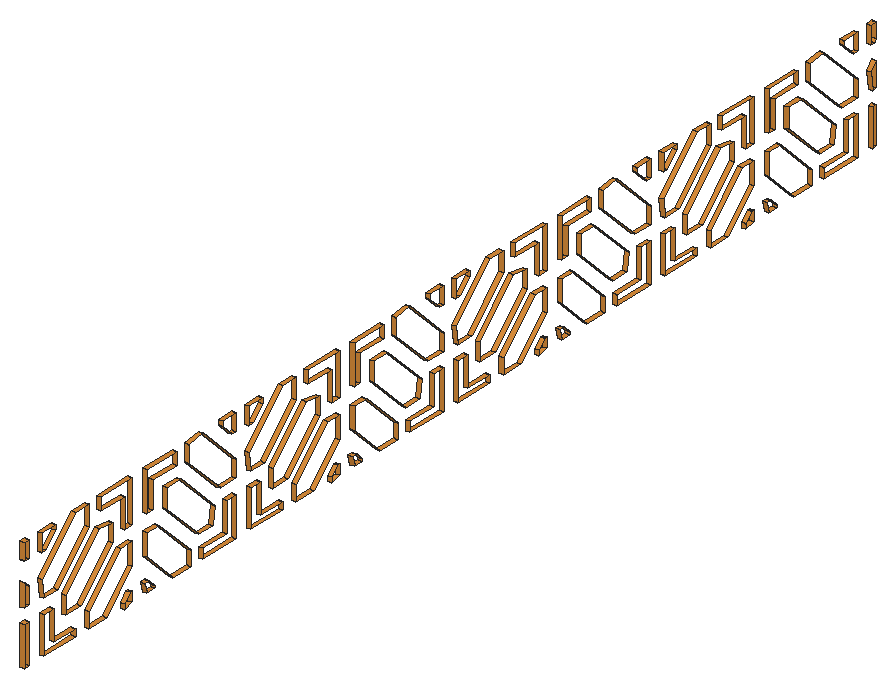
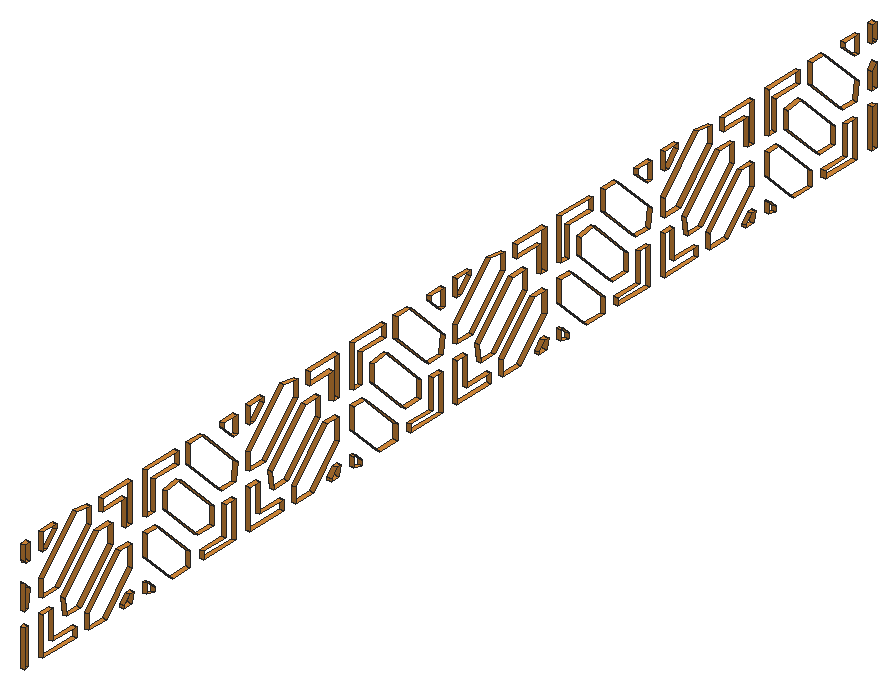
# SketchUp Ruby script. Lengths in inches.
U = 1.inch
M = Sketchup.active_model
def pt(a) = Geom::Point3d.new(a.map { |v| v * U })
def face(e, loops, mat)
  f = e.add_face(loops[0].map { |a| pt(a) })
  loops[1..].each { |l| e.add_face(l.map { |a| pt(a) }).erase! }
  f.material = f.back_material = mat if mat
  f
end
# faces: each face lists its corners as indices into pts; further lists are holes
def faces(e, pts, list, mat = nil) = list.each { |f| face(e, (f[0].is_a?(Array) ? f : [f]).map { |l| l.map { |i| pts[i] } }, mat) }
# xy, xz, yz: faces in a plane at the given z, y or x. An outline is a flat list of corners, or four numbers for a rectangle; further outlines are holes
def ring(l) = l.size == 4 ? [[l[0], l[1]], [l[2], l[1]], [l[2], l[3]], [l[0], l[3]]] : l.each_slice(2).to_a
def flat(e, list, mat, &to3) = list.each { |f| face(e, (f[0].is_a?(Array) ? f : [f]).map { |l| ring(l).map { |u, v| to3.(u, v) } }, mat) }
def xy(e, z, list, mat = nil) = flat(e, list, mat) { |x, y| [x, y, z] }
def xz(e, y, list, mat = nil) = flat(e, list, mat) { |x, z| [x, y, z] }
def yz(e, x, list, mat = nil) = flat(e, list, mat) { |y, z| [x, y, z] }
def lines(e, pts, list) = list.each { |a, b| e.add_line(pt(pts[a]), pt(pts[b])) }
# prism: a flat outline (further loops are holes) pulled along v
def prism(e, loops, v, mat = nil)
  f = face(e, loops, mat); d = Geom::Vector3d.new(v.map { |x| x * U })
  f.pushpull(f.normal.samedirection?(d) ? d.length : -d.length)
end
def box(e, o, s, mat = nil) = prism(e, [[o, [o[0] + s[0], o[1], o[2]], [o[0] + s[0], o[1] + s[1], o[2]], [o[0], o[1] + s[1], o[2]]]], [0, 0, s[2]], mat)
def at(x, y, z, deg = 0) = Geom::Transformation.translation(pt([x, y, z])) * Geom::Transformation.rotation(ORIGIN, Z_AXIS, deg.degrees)
def axes(o, x, y, z) = Geom::Transformation.new([*x, 0, *y, 0, *z, 0, *pt(o).to_a, 1])
def part(name) = M.definitions.add(name)
# library, detail: a bought-in or finely detailed component or shape, given as its bounding box
def library(name, o, s) = part(name).tap { |d| box(d.entities, o, s) }
def detail(e, o, s) = box(e.add_group.entities, o, s)
def put(e, d, t, mat = nil) = e.add_instance(d, t).tap { |i| i.material = mat if mat }
def group(e, t, mat = nil) = e.add_group.tap { |g| g.transformation = t; g.material = mat if mat }.entities
root = M.entities
M.materials.add("1056 AP 9903 Mellow Melon-N").color = [219, 142, 59]
xy(root,171.04,[[14.35,14.79,15.0625,15.84],[14.35,41.6875,15.0625,43.42],[14.35,47.3,15.0625,51.22],[14.35,53.82,15.0625,61.1875],[14.35,87.03,15.0625,88.76],
  [14.35,92.64,15.0625,96.56],[14.35,99.16,15.0625,106.53],[14.35,132.375,15.0625,134.11],[14.35,137.98,15.0625,141.91],[14.35,144.51,15.0625,151.875],
  [14.35,177.72,15.0625,179.45],[14.35,183.33,15.0625,187.25],[14.35,189.85,15.0625,197.22]],"1056 AP 9903 Mellow Melon-N")
xy(root,171.08,[[14.35,19.08,15.0625,25.95],[14.35,28.96,15.0625,32.8],[14.35,64.42,15.0625,71.3],[14.35,74.31,15.0625,78.15],[14.35,109.77,15.0625,116.64],
  [14.35,119.65,15.0625,123.49],[14.35,155.11,15.0625,161.99],[14.35,164.99,15.0625,168.84],[14.35,200.46,15.0625,201.3125]],"1056 AP 9903 Mellow Melon-N")
xy(root,172.375,[[14.35,21.23,15.0625,25.95],[14.35,66.57,15.0625,71.3],[14.35,111.92,15.0625,116.64],[14.35,157.26,15.0625,161.99]],"1056 AP 9903 Mellow Melon-N")
xy(root,172.76,[[14.35,41.25,15.0625,42.125],[14.35,53.82,15.0625,59.02],[14.35,86.6,15.0625,87.47],[14.35,99.16,15.0625,104.37],[14.35,131.94,15.0625,132.8125],
  [14.35,144.51,15.0625,149.71],[14.35,177.28,15.0625,178.16],[14.35,189.85,15.0625,195.05]],"1056 AP 9903 Mellow Melon-N")
xy(root,172.81,[[14.35,37.99,15.0625,38.41],[14.35,83.33,15.0625,83.76],[14.35,128.68,15.0625,129.1],[14.35,174.02,15.0625,174.45]],"1056 AP 9903 Mellow Melon-N")
xy(root,175.34,[[14.35,52.92,15.0625,55.99],[14.35,98.27,15.0625,101.33],[14.35,143.61,15.0625,146.68],[14.35,188.96,15.0625,192.02]],"1056 AP 9903 Mellow Melon-N")
xy(root,175.41,[[14.35,23.81,15.0625,27.21],[14.35,69.15,15.0625,72.56],[14.35,114.49,15.0625,117.9],[14.35,159.84,15.0625,163.24]],"1056 AP 9903 Mellow Melon-N")
xy(root,177.58,[[14.35,19.08,15.0625,21.23],[14.35,64.42,15.0625,66.57],[14.35,109.77,15.0625,111.92],[14.35,155.11,15.0625,157.26],[14.35,200.46,15.0625,201.3125]],"1056 AP 9903 Mellow Melon-N")
xy(root,177.92,[[14.35,14.79,15.0625,15.84],[14.35,59.02,15.0625,61.1875],[14.35,104.37,15.0625,106.53],[14.35,149.71,15.0625,151.875],[14.35,195.05,15.0625,197.22]],"1056 AP 9903 Mellow Melon-N")
xy(root,180.18,[[14.35,19.08,15.0625,22.06],[14.35,64.42,15.0625,67.4],[14.35,109.77,15.0625,112.75],[14.35,155.11,15.0625,158.09],[14.35,200.46,15.0625,201.3125]],"1056 AP 9903 Mellow Melon-N")
xy(root,180.49,[[14.35,14.79,15.0625,15.84],[14.35,41.6875,15.0625,44.32],[14.35,57.69,15.0625,61.1875],[14.35,87.03,15.0625,89.66],[14.35,103.04,15.0625,106.53],
  [14.35,132.375,15.0625,135],[14.35,148.38,15.0625,151.875],[14.35,177.72,15.0625,180.35],[14.35,193.72,15.0625,197.22]],"1056 AP 9903 Mellow Melon-N")
xy(root,180.61,[[14.35,35.87,15.0625,38.41],[14.35,81.21,15.0625,83.76],[14.35,126.55,15.0625,129.1],[14.35,171.9,15.0625,174.45]],"1056 AP 9903 Mellow Melon-N")
xy(root,183.21,[[14.35,36.7,15.0625,38.41],[14.35,82.04,15.0625,83.76],[14.35,127.38,15.0625,129.1],[14.35,172.73,15.0625,174.45]],"1056 AP 9903 Mellow Melon-N")
xy(root,183.5,[[14.35,41.6875,15.0625,42.99],[14.35,87.03,15.0625,88.33],[14.35,132.375,15.0625,133.67],[14.35,177.72,15.0625,179.02]],"1056 AP 9903 Mellow Melon-N")
xy(root,185.65,[[14.35,46.02,15.0625,49.09],[14.35,91.36,15.0625,94.43],[14.35,136.71,15.0625,139.77],[14.35,182.05,15.0625,185.12]],"1056 AP 9903 Mellow Melon-N")
xy(root,187.54,[[14.35,18.65,15.0625,19.5],[14.35,63.99,15.0625,64.84],[14.35,109.34,15.0625,110.1875],[14.35,154.68,15.0625,155.53],[14.35,200.03,15.0625,200.875]],"1056 AP 9903 Mellow Melon-N")
xy(root,187.8,[[14.35,14.97,15.0625,15.84],[14.35,60.3125,15.0625,61.1875],[14.35,105.66,15.0625,106.53],[14.35,151,15.0625,151.875],[14.35,196.34,15.0625,197.22]],"1056 AP 9903 Mellow Melon-N")
xy(root,188.23,[[14.35,42.99,15.0625,48.1875],[14.35,88.33,15.0625,93.53],[14.35,133.67,15.0625,138.875],[14.35,179.02,15.0625,184.22]],"1056 AP 9903 Mellow Melon-N")
xy(root,188.41,[[14.35,31.54,15.0625,36.7],[14.35,76.88,15.0625,82.04],[14.35,122.23,15.0625,127.38],[14.35,167.57,15.0625,172.73]],"1056 AP 9903 Mellow Melon-N")
xy(root,190.375,[[14.35,41.6875,15.0625,48.1875],[14.35,87.03,15.0625,93.53],[14.35,132.375,15.0625,138.875],[14.35,177.72,15.0625,184.22]],"1056 AP 9903 Mellow Melon-N")
xy(root,190.58,[[14.35,18.65,15.0625,21.66],[14.35,25.99,15.0625,28.96],[14.35,31.54,15.0625,38.41],[14.35,63.99,15.0625,67],[14.35,71.33,15.0625,74.31],
  [14.35,76.88,15.0625,83.76],[14.35,109.34,15.0625,112.35],[14.35,116.67,15.0625,119.65],[14.35,122.23,15.0625,129.1],[14.35,154.68,15.0625,157.6875],
  [14.35,162.02,15.0625,164.99],[14.35,167.57,15.0625,174.45],[14.35,200.03,15.0625,201.3125]],"1056 AP 9903 Mellow Melon-N")
xy(root,190.8,[[14.35,14.79,15.0625,15.84],[14.35,58.15,15.0625,61.1875],[14.35,103.5,15.0625,106.53],[14.35,148.84,15.0625,151.875],[14.35,194.1875,15.0625,197.22]],"1056 AP 9903 Mellow Melon-N")
xz(root,14.79,[[14.35,171.04,15.0625,177.92],[14.35,180.49,15.0625,184.53],[14.35,187.98,15.0625,190.8]],"1056 AP 9903 Mellow Melon-N")
xz(root,15.84,[[14.35,171.04,15.0625,177.92],[14.35,180.49,15.0625,183.47],[14.35,187.8,15.0625,190.8]],"1056 AP 9903 Mellow Melon-N")
xz(root,18.65,[[14.35,187.54,15.0625,190.58]],"1056 AP 9903 Mellow Melon-N")
xz(root,19.08,[[14.35,171.08,15.0625,177.58]],"1056 AP 9903 Mellow Melon-N")
xz(root,21.23,[[14.35,172.375,15.0625,177.58]],"1056 AP 9903 Mellow Melon-N")
xz(root,21.66,[[14.35,189.7,15.0625,190.58]],"1056 AP 9903 Mellow Melon-N")
xz(root,23.81,[[14.35,175.41,15.0625,178.47]],"1056 AP 9903 Mellow Melon-N")
xz(root,25.95,[[14.35,171.08,15.0625,172.375]],"1056 AP 9903 Mellow Melon-N")
xz(root,28.96,[[14.35,171.08,15.0625,173.71],[14.35,187.08,15.0625,190.58]],"1056 AP 9903 Mellow Melon-N")
xz(root,31.54,[[14.35,188.41,15.0625,190.58]],"1056 AP 9903 Mellow Melon-N")
xz(root,34.12,[[14.35,182.3125,15.0625,185.375]],"1056 AP 9903 Mellow Melon-N")
xz(root,36.7,[[14.35,170.64,15.0625,171.51],[14.35,183.21,15.0625,188.41]],"1056 AP 9903 Mellow Melon-N")
xz(root,38.41,[[14.35,171.08,15.0625,172.81],[14.35,176.68,15.0625,180.61],[14.35,183.21,15.0625,190.58]],"1056 AP 9903 Mellow Melon-N")
xz(root,41.6875,[[14.35,176.65,15.0625,180.49],[14.35,183.5,15.0625,190.375]],"1056 AP 9903 Mellow Melon-N")
xz(root,42.99,[[14.35,183.5,15.0625,188.23]],"1056 AP 9903 Mellow Melon-N")
xz(root,43.42,[[14.35,171.04,15.0625,171.47]],"1056 AP 9903 Mellow Melon-N")
xz(root,46.02,[[14.35,182.24,15.0625,185.65]],"1056 AP 9903 Mellow Melon-N")
xz(root,48.1875,[[14.35,188.23,15.0625,190.375]],"1056 AP 9903 Mellow Melon-N")
xz(root,50.79,[[14.35,187.4,15.0625,190.375]],"1056 AP 9903 Mellow Melon-N")
xz(root,51.22,[[14.35,171.04,15.0625,173.59]],"1056 AP 9903 Mellow Melon-N")
xz(root,53.82,[[14.35,171.04,15.0625,172.76]],"1056 AP 9903 Mellow Melon-N")
xz(root,58.15,[[14.35,189.95,15.0625,190.8]],"1056 AP 9903 Mellow Melon-N")
xz(root,59.02,[[14.35,172.76,15.0625,177.92]],"1056 AP 9903 Mellow Melon-N")
xz(root,61.1875,[[14.35,171.04,15.0625,177.92],[14.35,180.49,15.0625,183.47],[14.35,187.8,15.0625,190.8]],"1056 AP 9903 Mellow Melon-N")
xz(root,63.99,[[14.35,187.54,15.0625,190.58]],"1056 AP 9903 Mellow Melon-N")
xz(root,64.42,[[14.35,171.08,15.0625,177.58]],"1056 AP 9903 Mellow Melon-N")
xz(root,66.57,[[14.35,172.375,15.0625,177.58]],"1056 AP 9903 Mellow Melon-N")
xz(root,67,[[14.35,189.7,15.0625,190.58]],"1056 AP 9903 Mellow Melon-N")
xz(root,69.15,[[14.35,175.41,15.0625,178.47]],"1056 AP 9903 Mellow Melon-N")
xz(root,71.3,[[14.35,171.08,15.0625,172.375]],"1056 AP 9903 Mellow Melon-N")
xz(root,74.31,[[14.35,171.08,15.0625,173.71],[14.35,187.08,15.0625,190.58]],"1056 AP 9903 Mellow Melon-N")
xz(root,76.88,[[14.35,188.41,15.0625,190.58]],"1056 AP 9903 Mellow Melon-N")
xz(root,79.46,[[14.35,182.3125,15.0625,185.375]],"1056 AP 9903 Mellow Melon-N")
xz(root,82.04,[[14.35,170.64,15.0625,171.51],[14.35,183.21,15.0625,188.41]],"1056 AP 9903 Mellow Melon-N")
xz(root,83.76,[[14.35,171.08,15.0625,172.81],[14.35,176.68,15.0625,180.61],[14.35,183.21,15.0625,190.58]],"1056 AP 9903 Mellow Melon-N")
xz(root,87.03,[[14.35,176.65,15.0625,180.49],[14.35,183.5,15.0625,190.375]],"1056 AP 9903 Mellow Melon-N")
xz(root,88.33,[[14.35,183.5,15.0625,188.23]],"1056 AP 9903 Mellow Melon-N")
xz(root,88.76,[[14.35,171.04,15.0625,171.47]],"1056 AP 9903 Mellow Melon-N")
xz(root,91.36,[[14.35,182.24,15.0625,185.65]],"1056 AP 9903 Mellow Melon-N")
xz(root,93.53,[[14.35,188.23,15.0625,190.375]],"1056 AP 9903 Mellow Melon-N")
xz(root,96.13,[[14.35,187.4,15.0625,190.375]],"1056 AP 9903 Mellow Melon-N")
xz(root,96.56,[[14.35,171.04,15.0625,173.59]],"1056 AP 9903 Mellow Melon-N")
xz(root,99.16,[[14.35,171.04,15.0625,172.76]],"1056 AP 9903 Mellow Melon-N")
xz(root,103.5,[[14.35,189.95,15.0625,190.8]],"1056 AP 9903 Mellow Melon-N")
xz(root,104.37,[[14.35,172.76,15.0625,177.92]],"1056 AP 9903 Mellow Melon-N")
xz(root,106.53,[[14.35,171.04,15.0625,177.92],[14.35,180.49,15.0625,183.47],[14.35,187.8,15.0625,190.8]],"1056 AP 9903 Mellow Melon-N")
xz(root,109.34,[[14.35,187.54,15.0625,190.58]],"1056 AP 9903 Mellow Melon-N")
xz(root,109.77,[[14.35,171.08,15.0625,177.58]],"1056 AP 9903 Mellow Melon-N")
xz(root,111.92,[[14.35,172.375,15.0625,177.58]],"1056 AP 9903 Mellow Melon-N")
xz(root,112.35,[[14.35,189.7,15.0625,190.58]],"1056 AP 9903 Mellow Melon-N")
xz(root,114.49,[[14.35,175.41,15.0625,178.47]],"1056 AP 9903 Mellow Melon-N")
xz(root,116.64,[[14.35,171.08,15.0625,172.375]],"1056 AP 9903 Mellow Melon-N")
xz(root,119.65,[[14.35,171.08,15.0625,173.71],[14.35,187.08,15.0625,190.58]],"1056 AP 9903 Mellow Melon-N")
xz(root,122.23,[[14.35,188.41,15.0625,190.58]],"1056 AP 9903 Mellow Melon-N")
xz(root,124.81,[[14.35,182.3125,15.0625,185.375]],"1056 AP 9903 Mellow Melon-N")
xz(root,127.38,[[14.35,170.64,15.0625,171.51],[14.35,183.21,15.0625,188.41]],"1056 AP 9903 Mellow Melon-N")
xz(root,129.1,[[14.35,171.08,15.0625,172.81],[14.35,176.68,15.0625,180.61],[14.35,183.21,15.0625,190.58]],"1056 AP 9903 Mellow Melon-N")
xz(root,132.375,[[14.35,176.65,15.0625,180.49],[14.35,183.5,15.0625,190.375]],"1056 AP 9903 Mellow Melon-N")
xz(root,133.67,[[14.35,183.5,15.0625,188.23]],"1056 AP 9903 Mellow Melon-N")
xz(root,134.11,[[14.35,171.04,15.0625,171.47]],"1056 AP 9903 Mellow Melon-N")
xz(root,136.71,[[14.35,182.24,15.0625,185.65]],"1056 AP 9903 Mellow Melon-N")
xz(root,138.875,[[14.35,188.23,15.0625,190.375]],"1056 AP 9903 Mellow Melon-N")
xz(root,141.48,[[14.35,187.4,15.0625,190.375]],"1056 AP 9903 Mellow Melon-N")
xz(root,141.91,[[14.35,171.04,15.0625,173.59]],"1056 AP 9903 Mellow Melon-N")
xz(root,144.51,[[14.35,171.04,15.0625,172.76]],"1056 AP 9903 Mellow Melon-N")
xz(root,148.84,[[14.35,189.95,15.0625,190.8]],"1056 AP 9903 Mellow Melon-N")
xz(root,149.71,[[14.35,172.76,15.0625,177.92]],"1056 AP 9903 Mellow Melon-N")
xz(root,151.875,[[14.35,171.04,15.0625,177.92],[14.35,180.49,15.0625,183.47],[14.35,187.8,15.0625,190.8]],"1056 AP 9903 Mellow Melon-N")
xz(root,154.68,[[14.35,187.54,15.0625,190.58]],"1056 AP 9903 Mellow Melon-N")
xz(root,155.11,[[14.35,171.08,15.0625,177.58]],"1056 AP 9903 Mellow Melon-N")
xz(root,157.26,[[14.35,172.375,15.0625,177.58]],"1056 AP 9903 Mellow Melon-N")
xz(root,157.6875,[[14.35,189.7,15.0625,190.58]],"1056 AP 9903 Mellow Melon-N")
xz(root,159.84,[[14.35,175.41,15.0625,178.47]],"1056 AP 9903 Mellow Melon-N")
xz(root,161.99,[[14.35,171.08,15.0625,172.375]],"1056 AP 9903 Mellow Melon-N")
xz(root,164.99,[[14.35,171.08,15.0625,173.71],[14.35,187.08,15.0625,190.58]],"1056 AP 9903 Mellow Melon-N")
xz(root,167.57,[[14.35,188.41,15.0625,190.58]],"1056 AP 9903 Mellow Melon-N")
xz(root,170.15,[[14.35,182.3125,15.0625,185.375]],"1056 AP 9903 Mellow Melon-N")
xz(root,172.73,[[14.35,170.64,15.0625,171.51],[14.35,183.21,15.0625,188.41]],"1056 AP 9903 Mellow Melon-N")
xz(root,174.45,[[14.35,171.08,15.0625,172.81],[14.35,176.68,15.0625,180.61],[14.35,183.21,15.0625,190.58]],"1056 AP 9903 Mellow Melon-N")
xz(root,177.72,[[14.35,176.65,15.0625,180.49],[14.35,183.5,15.0625,190.375]],"1056 AP 9903 Mellow Melon-N")
xz(root,179.02,[[14.35,183.5,15.0625,188.23]],"1056 AP 9903 Mellow Melon-N")
xz(root,179.45,[[14.35,171.04,15.0625,171.47]],"1056 AP 9903 Mellow Melon-N")
xz(root,182.05,[[14.35,182.24,15.0625,185.65]],"1056 AP 9903 Mellow Melon-N")
xz(root,184.22,[[14.35,188.23,15.0625,190.375]],"1056 AP 9903 Mellow Melon-N")
xz(root,186.82,[[14.35,187.4,15.0625,190.375]],"1056 AP 9903 Mellow Melon-N")
xz(root,187.25,[[14.35,171.04,15.0625,173.59]],"1056 AP 9903 Mellow Melon-N")
xz(root,189.85,[[14.35,171.04,15.0625,172.76]],"1056 AP 9903 Mellow Melon-N")
xz(root,194.1875,[[14.35,189.95,15.0625,190.8]],"1056 AP 9903 Mellow Melon-N")
xz(root,195.05,[[14.35,172.76,15.0625,177.92]],"1056 AP 9903 Mellow Melon-N")
xz(root,197.22,[[14.35,171.04,15.0625,177.92],[14.35,180.49,15.0625,183.47],[14.35,187.8,15.0625,190.8]],"1056 AP 9903 Mellow Melon-N")
xz(root,200.03,[[14.35,187.54,15.0625,190.58]],"1056 AP 9903 Mellow Melon-N")
xz(root,200.46,[[14.35,171.08,15.0625,177.58]],"1056 AP 9903 Mellow Melon-N")
xz(root,201.3125,[[14.35,171.08,15.0625,177.58],[14.35,180.18,15.0625,184.53],[14.35,187.98,15.0625,190.58]],"1056 AP 9903 Mellow Melon-N")
p = [[15.0625,36.7,170.64],[15.0625,38.41,171.08],[14.35,38.41,171.08],[14.35,36.7,170.64],[15.0625,82.04,170.64],[15.0625,83.76,171.08],
  [14.35,83.76,171.08],[14.35,82.04,170.64],[15.0625,127.38,170.64],[15.0625,129.1,171.08],[14.35,129.1,171.08],[14.35,127.38,170.64],
  [15.0625,172.73,170.64],[15.0625,174.45,171.08],[14.35,174.45,171.08],[14.35,172.73,170.64],[15.0625,41.25,172.76],[15.0625,41.6875,171.04],
  [14.35,41.6875,171.04],[14.35,41.25,172.76],[15.0625,41.6875,176.65],[15.0625,47.3,171.04],[14.35,47.3,171.04],[14.35,41.6875,176.65],
  [15.0625,86.6,172.76],[15.0625,87.03,171.04],[14.35,87.03,171.04],[14.35,86.6,172.76],[15.0625,87.03,176.65],[15.0625,92.64,171.04],
  [14.35,92.64,171.04],[14.35,87.03,176.65],[15.0625,131.94,172.76],[15.0625,132.375,171.04],[14.35,132.375,171.04],[14.35,131.94,172.76],
  [15.0625,132.375,176.65],[15.0625,137.98,171.04],[14.35,137.98,171.04],[14.35,132.375,176.65],[15.0625,177.28,172.76],[15.0625,177.72,171.04],
  [14.35,177.72,171.04],[14.35,177.28,172.76],[15.0625,177.72,176.65],[15.0625,183.33,171.04],[14.35,183.33,171.04],[14.35,177.72,176.65],
  [15.0625,32.8,171.08],[15.0625,38.41,176.68],[14.35,38.41,176.68],[14.35,32.8,171.08],[15.0625,78.15,171.08],[15.0625,83.76,176.68],
  [14.35,83.76,176.68],[14.35,78.15,171.08],[15.0625,123.49,171.08],[15.0625,129.1,176.68],[14.35,129.1,176.68],[14.35,123.49,171.08],
  [15.0625,168.84,171.08],[15.0625,174.45,176.68],[14.35,174.45,176.68],[14.35,168.84,171.08],[15.0625,37.99,172.81],[15.0625,36.7,171.51],
  [14.35,36.7,171.51],[14.35,37.99,172.81],[15.0625,43.42,171.47],[15.0625,42.125,172.76],[14.35,42.125,172.76],[14.35,43.42,171.47],
  [15.0625,83.33,172.81],[15.0625,82.04,171.51],[14.35,82.04,171.51],[14.35,83.33,172.81],[15.0625,88.76,171.47],[15.0625,87.47,172.76],
  [14.35,87.47,172.76],[14.35,88.76,171.47],[15.0625,128.68,172.81],[15.0625,127.38,171.51],[14.35,127.38,171.51],[14.35,128.68,172.81],
  [15.0625,134.11,171.47],[15.0625,132.8125,172.76],[14.35,132.8125,172.76],[14.35,134.11,171.47],[15.0625,174.02,172.81],[15.0625,172.73,171.51],
  [14.35,172.73,171.51],[14.35,174.02,172.81],[15.0625,179.45,171.47],[15.0625,178.16,172.76],[14.35,178.16,172.76],[14.35,179.45,171.47],
  [15.0625,51.22,173.59],[15.0625,44.32,180.49],[14.35,44.32,180.49],[14.35,51.22,173.59],[15.0625,96.56,173.59],[15.0625,89.66,180.49],
  [14.35,89.66,180.49],[14.35,96.56,173.59],[15.0625,141.91,173.59],[15.0625,135,180.49],[14.35,135,180.49],[14.35,141.91,173.59],
  [15.0625,187.25,173.59],[15.0625,180.35,180.49],[14.35,180.35,180.49],[14.35,187.25,173.59],[15.0625,35.87,180.61],[15.0625,28.96,173.71],
  [14.35,28.96,173.71],[14.35,35.87,180.61],[15.0625,81.21,180.61],[15.0625,74.31,173.71],[14.35,74.31,173.71],[14.35,81.21,180.61],
  [15.0625,126.55,180.61],[15.0625,119.65,173.71],[14.35,119.65,173.71],[14.35,126.55,180.61],[15.0625,171.9,180.61],[15.0625,164.99,173.71],
  [14.35,164.99,173.71],[14.35,171.9,180.61],[15.0625,46.02,182.24],[15.0625,52.92,175.34],[14.35,52.92,175.34],[14.35,46.02,182.24],
  [15.0625,55.99,175.34],[15.0625,56.42,178.32],[14.35,56.42,178.32],[14.35,55.99,175.34],[15.0625,91.36,182.24],[15.0625,98.27,175.34],
  [14.35,98.27,175.34],[14.35,91.36,182.24],[15.0625,101.33,175.34],[15.0625,101.76,178.32],[14.35,101.76,178.32],[14.35,101.33,175.34],
  [15.0625,136.71,182.24],[15.0625,143.61,175.34],[14.35,143.61,175.34],[14.35,136.71,182.24],[15.0625,146.68,175.34],[15.0625,147.1,178.32],
  [14.35,147.1,178.32],[14.35,146.68,175.34],[15.0625,182.05,182.24],[15.0625,188.96,175.34],[14.35,188.96,175.34],[14.35,182.05,182.24],
  [15.0625,192.02,175.34],[15.0625,192.45,178.32],[14.35,192.45,178.32],[14.35,192.02,175.34],[15.0625,27.21,175.41],[15.0625,34.12,182.3125],
  [14.35,34.12,182.3125],[14.35,27.21,175.41],[15.0625,72.56,175.41],[15.0625,79.46,182.3125],[14.35,79.46,182.3125],[14.35,72.56,175.41],
  [15.0625,117.9,175.41],[15.0625,124.81,182.3125],[14.35,124.81,182.3125],[14.35,117.9,175.41],[15.0625,163.24,175.41],[15.0625,170.15,182.3125],
  [14.35,170.15,182.3125],[14.35,163.24,175.41],[15.0625,49.09,185.65],[14.35,49.09,185.65],[15.0625,94.43,185.65],[14.35,94.43,185.65],
  [15.0625,139.77,185.65],[14.35,139.77,185.65],[15.0625,185.12,185.65],[14.35,185.12,185.65],[15.0625,31.14,185.81],[15.0625,23.81,178.47],
  [14.35,23.81,178.47],[14.35,31.14,185.81],[15.0625,76.48,185.81],[15.0625,69.15,178.47],[14.35,69.15,178.47],[14.35,76.48,185.81],
  [15.0625,121.83,185.81],[15.0625,114.49,178.47],[14.35,114.49,178.47],[14.35,121.83,185.81],[15.0625,167.17,185.81],[15.0625,159.84,178.47],
  [14.35,159.84,178.47],[14.35,167.17,185.81],[15.0625,18.65,183.24],[15.0625,19.08,180.18],[14.35,19.08,180.18],[14.35,18.65,183.24],
  [15.0625,22.06,180.18],[15.0625,28.96,187.08],[14.35,28.96,187.08],[14.35,22.06,180.18],[15.0625,63.99,183.24],[15.0625,64.42,180.18],
  [14.35,64.42,180.18],[14.35,63.99,183.24],[15.0625,67.4,180.18],[15.0625,74.31,187.08],[14.35,74.31,187.08],[14.35,67.4,180.18],
  [15.0625,109.33,183.24],[15.0625,109.77,180.18],[14.35,109.77,180.18],[14.35,109.33,183.24],[15.0625,112.75,180.18],[15.0625,119.65,187.08],
  [14.35,119.65,187.08],[14.35,112.75,180.18],[15.0625,154.68,183.24],[15.0625,155.11,180.18],[14.35,155.11,180.18],[14.35,154.68,183.24],
  [15.0625,158.09,180.18],[15.0625,164.99,187.08],[14.35,164.99,187.08],[14.35,158.09,180.18],[15.0625,200.02,183.24],[15.0625,200.46,180.18],
  [14.35,200.46,180.18],[14.35,200.02,183.24],[15.0625,50.79,187.4],[15.0625,57.69,180.49],[14.35,57.69,180.49],[14.35,50.79,187.4],
  [15.0625,96.13,187.4],[15.0625,103.04,180.49],[14.35,103.04,180.49],[14.35,96.13,187.4],[15.0625,141.48,187.4],[15.0625,148.38,180.49],
  [14.35,148.38,180.49],[14.35,141.48,187.4],[15.0625,186.82,187.4],[15.0625,193.72,180.49],[14.35,193.72,180.49],[14.35,186.82,187.4],
  [15.0625,25.99,190.58],[14.35,25.99,190.58],[15.0625,71.33,190.58],[14.35,71.33,190.58],[15.0625,116.67,190.58],[14.35,116.67,190.58],
  [15.0625,162.02,190.58],[14.35,162.02,190.58],[15.0625,201.3125,184.53],[14.35,201.3125,184.53],[15.0625,15.84,183.47],[15.0625,14.79,184.53],
  [14.35,14.79,184.53],[14.35,15.84,183.47],[15.0625,61.1875,183.47],[15.0625,53.85,190.81],[14.35,53.85,190.81],[14.35,61.1875,183.47],
  [15.0625,106.53,183.47],[15.0625,99.19,190.81],[14.35,99.19,190.81],[14.35,106.53,183.47],[15.0625,151.875,183.47],[15.0625,144.54,190.81],
  [14.35,144.54,190.81],[14.35,151.875,183.47],[15.0625,197.22,183.47],[15.0625,189.88,190.81],[14.35,189.88,190.81],[14.35,197.22,183.47],
  [15.0625,34.12,185.375],[14.35,34.12,185.375],[15.0625,79.46,185.375],[14.35,79.46,185.375],[15.0625,124.81,185.375],[14.35,124.81,185.375],
  [15.0625,170.15,185.375],[14.35,170.15,185.375],[15.0625,19.5,187.54],[15.0625,21.66,189.7],[14.35,21.66,189.7],[14.35,19.5,187.54],
  [15.0625,64.84,187.54],[15.0625,67,189.7],[14.35,67,189.7],[14.35,64.84,187.54],[15.0625,110.1875,187.54],[15.0625,112.35,189.7],
  [14.35,112.35,189.7],[14.35,110.1875,187.54],[15.0625,155.53,187.54],[15.0625,157.6875,189.7],[14.35,157.6875,189.7],[14.35,155.53,187.54],
  [15.0625,200.875,187.54],[15.0625,201.3125,187.98],[14.35,201.3125,187.98],[14.35,200.875,187.54],[15.0625,14.79,187.98],[15.0625,14.97,187.8],
  [14.35,14.97,187.8],[14.35,14.79,187.98],[15.0625,58.15,189.95],[15.0625,60.3125,187.8],[14.35,60.3125,187.8],[14.35,58.15,189.95],
  [15.0625,103.5,189.95],[15.0625,105.66,187.8],[14.35,105.66,187.8],[14.35,103.5,189.95],[15.0625,148.84,189.95],[15.0625,151,187.8],
  [14.35,151,187.8],[14.35,148.84,189.95],[15.0625,194.1875,189.95],[15.0625,196.34,187.8],[14.35,196.34,187.8],[14.35,194.1875,189.95],
  [15.0625,50.79,190.375],[14.35,50.79,190.375],[15.0625,96.13,190.375],[14.35,96.13,190.375],[15.0625,141.48,190.375],[14.35,141.48,190.375],
  [15.0625,186.82,190.375],[14.35,186.82,190.375]]
faces(root,p,[[0,1,2,3],[4,5,6,7],[8,9,10,11],[12,13,14,15],[16,17,18,19],[20,21,22,23],[24,25,26,27],[28,29,30,31],
  [32,33,34,35],[36,37,38,39],[40,41,42,43],[44,45,46,47],[48,49,50,51],[52,53,54,55],[56,57,58,59],[60,61,62,63],
  [64,65,66,67],[68,69,70,71],[72,73,74,75],[76,77,78,79],[80,81,82,83],[84,85,86,87],[88,89,90,91],[92,93,94,95],
  [96,97,98,99],[100,101,102,103],[104,105,106,107],[108,109,110,111],[112,113,114,115],[116,117,118,119],[120,121,122,123],[124,125,126,127],
  [128,129,130,131],[132,133,134,135],[136,137,138,139],[140,141,142,143],[144,145,146,147],[148,149,150,151],[152,153,154,155],[156,157,158,159],
  [160,161,162,163],[164,165,166,167],[168,169,170,171],[172,173,174,175],[133,176,177,134],[141,178,179,142],[149,180,181,150],[157,182,183,158],
  [184,185,186,187],[188,189,190,191],[192,193,194,195],[196,197,198,199],[200,201,202,203],[204,205,206,207],[208,209,210,211],[212,213,214,215],
  [216,217,218,219],[220,221,222,223],[224,225,226,227],[228,229,230,231],[232,233,234,235],[236,237,238,239],[240,241,242,243],[244,245,246,247],
  [248,249,250,251],[252,200,203,253],[254,208,211,255],[256,216,219,257],[258,224,227,259],[260,232,235,261],[262,263,264,265],[266,267,268,269],
  [270,271,272,273],[274,275,276,277],[278,279,280,281],[282,184,187,283],[284,188,191,285],[286,192,195,287],[288,196,199,289],[290,291,292,293],
  [294,295,296,297],[298,299,300,301],[302,303,304,305],[306,307,308,309],[310,311,312,313],[314,315,316,317],[318,319,320,321],[322,323,324,325],
  [326,327,328,329],[267,330,331,268],[271,332,333,272],[275,334,335,276],[279,336,337,280]],"1056 AP 9903 Mellow Melon-N")
